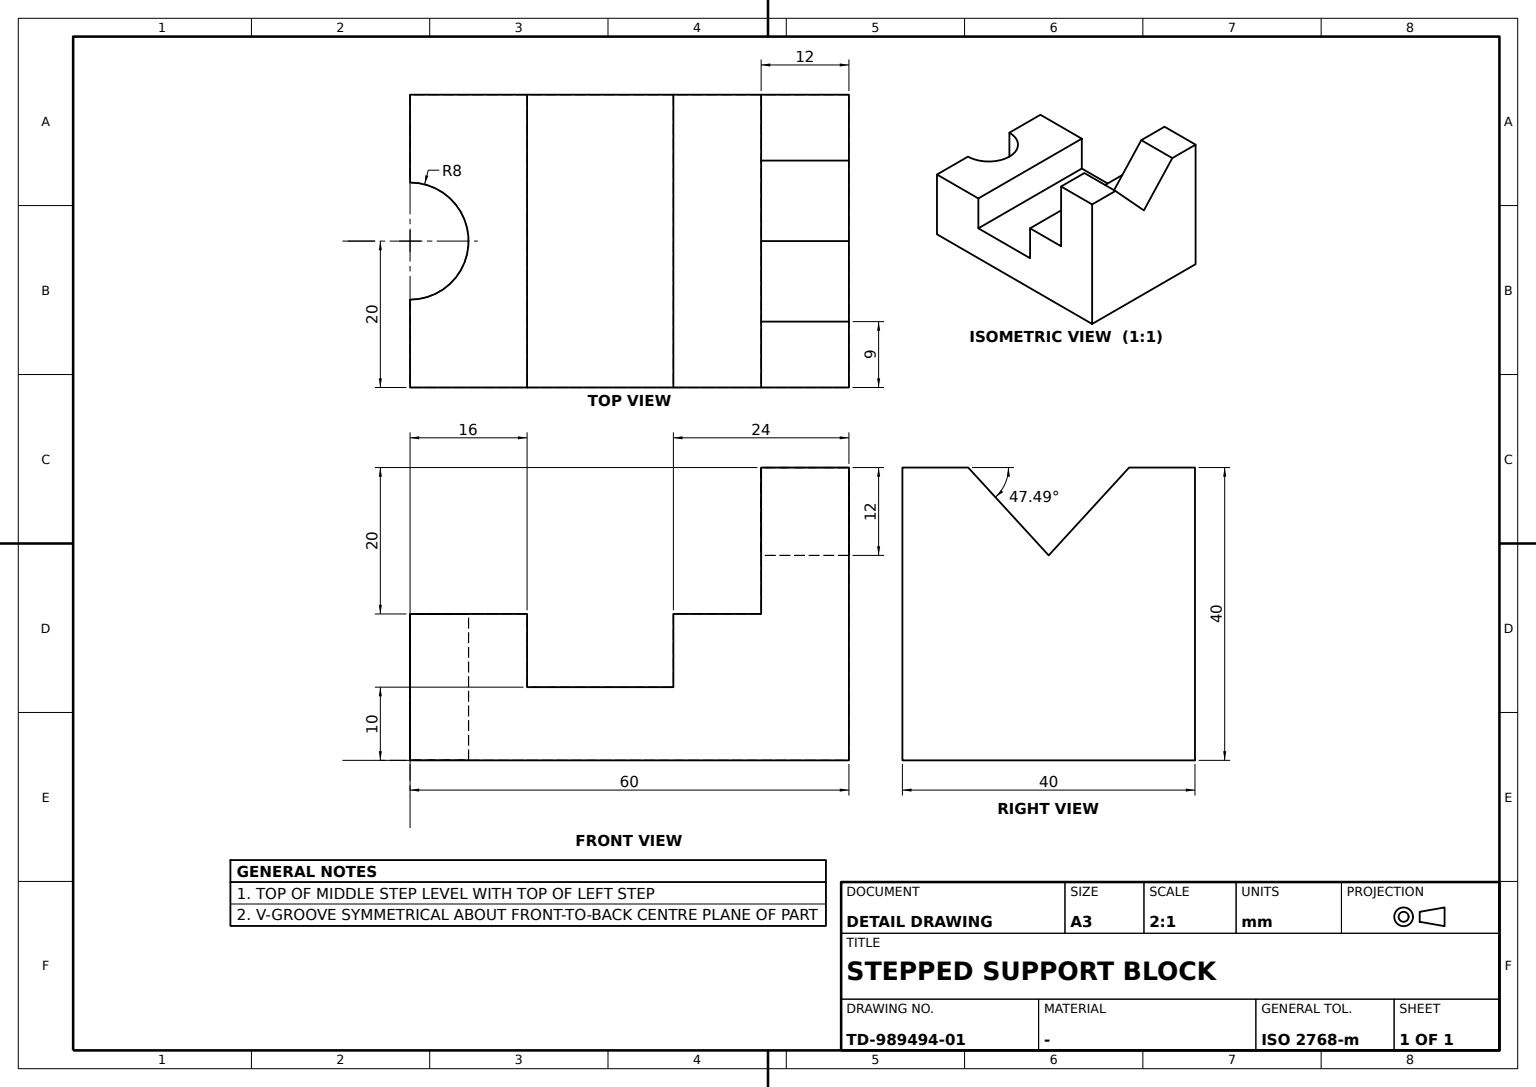
ISO-10303-21;
HEADER;
FILE_DESCRIPTION((''),'2;1');
FILE_NAME('','',(''),(''),'','','');
FILE_SCHEMA(('AUTOMOTIVE_DESIGN'));
ENDSEC;
DATA;
#1=APPLICATION_CONTEXT('');
#2=PRODUCT_CONTEXT('',#1,'mechanical');
#3=PRODUCT('','','',(#2));
#4=PRODUCT_DEFINITION_FORMATION('','',#3);
#5=PRODUCT_DEFINITION_CONTEXT('',#1,'design');
#6=PRODUCT_DEFINITION('','',#4,#5);
#7=PRODUCT_DEFINITION_SHAPE('','',#6);
#8=(LENGTH_UNIT()NAMED_UNIT(*)SI_UNIT(.MILLI.,.METRE.));
#9=(NAMED_UNIT(*)PLANE_ANGLE_UNIT()SI_UNIT($,.RADIAN.));
#10=(NAMED_UNIT(*)SI_UNIT($,.STERADIAN.)SOLID_ANGLE_UNIT());
#11=UNCERTAINTY_MEASURE_WITH_UNIT(LENGTH_MEASURE(0.005),#8,'distance_accuracy_value','');
#12=(GEOMETRIC_REPRESENTATION_CONTEXT(3)GLOBAL_UNCERTAINTY_ASSIGNED_CONTEXT((#11))GLOBAL_UNIT_ASSIGNED_CONTEXT((#8,#9,#10))REPRESENTATION_CONTEXT('',''));
#13=CARTESIAN_POINT('',(8.,0.,0.));
#14=VERTEX_POINT('',#13);
#15=CARTESIAN_POINT('',(20.,0.,0.));
#16=VERTEX_POINT('',#15);
#17=CARTESIAN_POINT('',(0.,0.,0.));
#18=DIRECTION('',(1.,0.,0.));
#19=VECTOR('',#18,1000.);
#20=LINE('',#17,#19);
#21=EDGE_CURVE('',#14,#16,#20,.T.);
#22=ORIENTED_EDGE('',*,*,#21,.T.);
#23=CARTESIAN_POINT('',(20.,0.,20.));
#24=VERTEX_POINT('',#23);
#25=DIRECTION('',(0.,0.,1.));
#26=VECTOR('',#25,1000.);
#27=LINE('',#15,#26);
#28=EDGE_CURVE('',#16,#24,#27,.T.);
#29=ORIENTED_EDGE('',*,*,#28,.T.);
#30=CARTESIAN_POINT('',(8.,0.,20.));
#31=VERTEX_POINT('',#30);
#32=CARTESIAN_POINT('',(0.,0.,20.));
#33=LINE('',#32,#19);
#34=EDGE_CURVE('',#31,#24,#33,.T.);
#35=ORIENTED_EDGE('',*,*,#34,.F.);
#36=LINE('',#13,#26);
#37=EDGE_CURVE('',#31,#14,#36,.F.);
#38=ORIENTED_EDGE('',*,*,#37,.T.);
#39=EDGE_LOOP('',(#22,#29,#35,#38));
#40=FACE_BOUND('',#39,.T.);
#41=DIRECTION('',(0.,1.,0.));
#42=AXIS2_PLACEMENT_3D('',#17,#41,#25);
#43=PLANE('',#42);
#44=ADVANCED_FACE('',(#40),#43,.F.);
#45=CARTESIAN_POINT('',(-8.,0.,20.));
#46=VERTEX_POINT('',#45);
#47=DIRECTION('',(0.,0.,-1.));
#48=DIRECTION('',(-1.,0.,0.));
#49=AXIS2_PLACEMENT_3D('',#32,#47,#48);
#50=CIRCLE('',#49,8.);
#51=EDGE_CURVE('',#31,#46,#50,.F.);
#52=ORIENTED_EDGE('',*,*,#51,.F.);
#53=ORIENTED_EDGE('',*,*,#34,.T.);
#54=CARTESIAN_POINT('',(20.,16.,20.));
#55=VERTEX_POINT('',#54);
#56=VECTOR('',#41,1000.);
#57=LINE('',#23,#56);
#58=EDGE_CURVE('',#24,#55,#57,.T.);
#59=ORIENTED_EDGE('',*,*,#58,.T.);
#60=CARTESIAN_POINT('',(-20.,16.,20.));
#61=VERTEX_POINT('',#60);
#62=CARTESIAN_POINT('',(0.,16.,20.));
#63=LINE('',#62,#19);
#64=EDGE_CURVE('',#61,#55,#63,.T.);
#65=ORIENTED_EDGE('',*,*,#64,.F.);
#66=CARTESIAN_POINT('',(-20.,0.,20.));
#67=VERTEX_POINT('',#66);
#68=LINE('',#66,#56);
#69=EDGE_CURVE('',#67,#61,#68,.T.);
#70=ORIENTED_EDGE('',*,*,#69,.F.);
#71=EDGE_CURVE('',#67,#46,#33,.T.);
#72=ORIENTED_EDGE('',*,*,#71,.T.);
#73=EDGE_LOOP('',(#52,#53,#59,#65,#70,#72));
#74=FACE_BOUND('',#73,.T.);
#75=CARTESIAN_POINT('',(0.,36.,20.));
#76=AXIS2_PLACEMENT_3D('',#75,#47,#41);
#77=PLANE('',#76);
#78=ADVANCED_FACE('',(#74),#77,.F.);
#79=CARTESIAN_POINT('',(-20.,16.,10.));
#80=VERTEX_POINT('',#79);
#81=CARTESIAN_POINT('',(20.,16.,10.));
#82=VERTEX_POINT('',#81);
#83=CARTESIAN_POINT('',(0.,16.,10.));
#84=LINE('',#83,#19);
#85=EDGE_CURVE('',#80,#82,#84,.T.);
#86=ORIENTED_EDGE('',*,*,#85,.F.);
#87=CARTESIAN_POINT('',(-20.,16.,0.));
#88=VECTOR('',#47,1000.);
#89=LINE('',#87,#88);
#90=EDGE_CURVE('',#61,#80,#89,.T.);
#91=ORIENTED_EDGE('',*,*,#90,.F.);
#92=ORIENTED_EDGE('',*,*,#64,.T.);
#93=CARTESIAN_POINT('',(20.,16.,0.));
#94=LINE('',#93,#88);
#95=EDGE_CURVE('',#55,#82,#94,.T.);
#96=ORIENTED_EDGE('',*,*,#95,.T.);
#97=EDGE_LOOP('',(#86,#91,#92,#96));
#98=FACE_BOUND('',#97,.T.);
#99=DIRECTION('',(0.,-1.,0.));
#100=AXIS2_PLACEMENT_3D('',#62,#99,#47);
#101=PLANE('',#100);
#102=ADVANCED_FACE('',(#98),#101,.F.);
#103=CARTESIAN_POINT('',(-20.,60.,0.));
#104=VERTEX_POINT('',#103);
#105=CARTESIAN_POINT('',(20.,60.,0.));
#106=VERTEX_POINT('',#105);
#107=CARTESIAN_POINT('',(0.,60.,0.));
#108=LINE('',#107,#19);
#109=EDGE_CURVE('',#104,#106,#108,.T.);
#110=ORIENTED_EDGE('',*,*,#109,.T.);
#111=VECTOR('',#99,1000.);
#112=LINE('',#15,#111);
#113=EDGE_CURVE('',#106,#16,#112,.T.);
#114=ORIENTED_EDGE('',*,*,#113,.T.);
#115=ORIENTED_EDGE('',*,*,#21,.F.);
#116=CARTESIAN_POINT('',(-8.,0.,0.));
#117=VERTEX_POINT('',#116);
#118=AXIS2_PLACEMENT_3D('',#17,#25,#18);
#119=CIRCLE('',#118,8.);
#120=EDGE_CURVE('',#14,#117,#119,.T.);
#121=ORIENTED_EDGE('',*,*,#120,.T.);
#122=CARTESIAN_POINT('',(-20.,0.,0.));
#123=VERTEX_POINT('',#122);
#124=EDGE_CURVE('',#123,#117,#20,.T.);
#125=ORIENTED_EDGE('',*,*,#124,.F.);
#126=LINE('',#122,#111);
#127=EDGE_CURVE('',#104,#123,#126,.T.);
#128=ORIENTED_EDGE('',*,*,#127,.F.);
#129=EDGE_LOOP('',(#110,#114,#115,#121,#125,#128));
#130=FACE_BOUND('',#129,.T.);
#131=AXIS2_PLACEMENT_3D('',#107,#25,#99);
#132=PLANE('',#131);
#133=ADVANCED_FACE('',(#130),#132,.F.);
#134=LINE('',#116,#26);
#135=EDGE_CURVE('',#117,#46,#134,.T.);
#136=ORIENTED_EDGE('',*,*,#135,.T.);
#137=ORIENTED_EDGE('',*,*,#71,.F.);
#138=LINE('',#122,#26);
#139=EDGE_CURVE('',#123,#67,#138,.T.);
#140=ORIENTED_EDGE('',*,*,#139,.F.);
#141=ORIENTED_EDGE('',*,*,#124,.T.);
#142=EDGE_LOOP('',(#136,#137,#140,#141));
#143=FACE_BOUND('',#142,.T.);
#144=ADVANCED_FACE('',(#143),#43,.F.);
#145=CARTESIAN_POINT('',(11.,60.,40.));
#146=VERTEX_POINT('',#145);
#147=CARTESIAN_POINT('',(11.,48.,40.));
#148=VERTEX_POINT('',#147);
#149=LINE('',#145,#111);
#150=EDGE_CURVE('',#146,#148,#149,.T.);
#151=ORIENTED_EDGE('',*,*,#150,.F.);
#152=CARTESIAN_POINT('',(0.,60.,28.));
#153=VERTEX_POINT('',#152);
#154=CARTESIAN_POINT('',(5.977358,60.,34.520755));
#155=DIRECTION('',(-0.675724629,0.,-0.73715414));
#156=VECTOR('',#155,1000.);
#157=LINE('',#154,#156);
#158=EDGE_CURVE('',#146,#153,#157,.T.);
#159=ORIENTED_EDGE('',*,*,#158,.T.);
#160=CARTESIAN_POINT('',(0.,48.,28.));
#161=VERTEX_POINT('',#160);
#162=LINE('',#152,#111);
#163=EDGE_CURVE('',#153,#161,#162,.T.);
#164=ORIENTED_EDGE('',*,*,#163,.T.);
#165=LINE('',#147,#156);
#166=EDGE_CURVE('',#148,#161,#165,.T.);
#167=ORIENTED_EDGE('',*,*,#166,.F.);
#168=EDGE_LOOP('',(#151,#159,#164,#167));
#169=FACE_BOUND('',#168,.T.);
#170=DIRECTION('',(-0.73715414,0.,0.675724629));
#171=AXIS2_PLACEMENT_3D('',#145,#170,#155);
#172=PLANE('',#171);
#173=ADVANCED_FACE('',(#169),#172,.T.);
#174=CARTESIAN_POINT('',(-20.,48.,40.));
#175=VERTEX_POINT('',#174);
#176=CARTESIAN_POINT('',(-20.,60.,40.));
#177=VERTEX_POINT('',#176);
#178=CARTESIAN_POINT('',(-20.,0.,40.));
#179=LINE('',#178,#56);
#180=EDGE_CURVE('',#175,#177,#179,.T.);
#181=ORIENTED_EDGE('',*,*,#180,.T.);
#182=LINE('',#103,#88);
#183=EDGE_CURVE('',#177,#104,#182,.T.);
#184=ORIENTED_EDGE('',*,*,#183,.T.);
#185=ORIENTED_EDGE('',*,*,#127,.T.);
#186=ORIENTED_EDGE('',*,*,#139,.T.);
#187=ORIENTED_EDGE('',*,*,#69,.T.);
#188=ORIENTED_EDGE('',*,*,#90,.T.);
#189=CARTESIAN_POINT('',(-20.,36.,10.));
#190=VERTEX_POINT('',#189);
#191=CARTESIAN_POINT('',(-20.,0.,10.));
#192=LINE('',#191,#56);
#193=EDGE_CURVE('',#80,#190,#192,.T.);
#194=ORIENTED_EDGE('',*,*,#193,.T.);
#195=CARTESIAN_POINT('',(-20.,36.,20.));
#196=VERTEX_POINT('',#195);
#197=CARTESIAN_POINT('',(-20.,36.,0.));
#198=LINE('',#197,#26);
#199=EDGE_CURVE('',#190,#196,#198,.T.);
#200=ORIENTED_EDGE('',*,*,#199,.T.);
#201=CARTESIAN_POINT('',(-20.,48.,20.));
#202=VERTEX_POINT('',#201);
#203=EDGE_CURVE('',#196,#202,#68,.T.);
#204=ORIENTED_EDGE('',*,*,#203,.T.);
#205=CARTESIAN_POINT('',(-20.,48.,0.));
#206=LINE('',#205,#26);
#207=EDGE_CURVE('',#202,#175,#206,.T.);
#208=ORIENTED_EDGE('',*,*,#207,.T.);
#209=EDGE_LOOP('',(#181,#184,#185,#186,#187,#188,#194,#200,#204,#208));
#210=FACE_BOUND('',#209,.T.);
#211=AXIS2_PLACEMENT_3D('',#122,#18,#41);
#212=PLANE('',#211);
#213=ADVANCED_FACE('',(#210),#212,.F.);
#214=ORIENTED_EDGE('',*,*,#199,.F.);
#215=CARTESIAN_POINT('',(20.,36.,10.));
#216=VERTEX_POINT('',#215);
#217=CARTESIAN_POINT('',(0.,36.,10.));
#218=LINE('',#217,#19);
#219=EDGE_CURVE('',#190,#216,#218,.T.);
#220=ORIENTED_EDGE('',*,*,#219,.T.);
#221=CARTESIAN_POINT('',(20.,36.,20.));
#222=VERTEX_POINT('',#221);
#223=CARTESIAN_POINT('',(20.,36.,0.));
#224=LINE('',#223,#26);
#225=EDGE_CURVE('',#216,#222,#224,.T.);
#226=ORIENTED_EDGE('',*,*,#225,.T.);
#227=LINE('',#75,#19);
#228=EDGE_CURVE('',#196,#222,#227,.T.);
#229=ORIENTED_EDGE('',*,*,#228,.F.);
#230=EDGE_LOOP('',(#214,#220,#226,#229));
#231=FACE_BOUND('',#230,.T.);
#232=AXIS2_PLACEMENT_3D('',#217,#41,#25);
#233=PLANE('',#232);
#234=ADVANCED_FACE('',(#231),#233,.F.);
#235=ORIENTED_EDGE('',*,*,#109,.F.);
#236=ORIENTED_EDGE('',*,*,#183,.F.);
#237=CARTESIAN_POINT('',(-11.,60.,40.));
#238=VERTEX_POINT('',#237);
#239=CARTESIAN_POINT('',(0.,60.,40.));
#240=LINE('',#239,#19);
#241=EDGE_CURVE('',#177,#238,#240,.T.);
#242=ORIENTED_EDGE('',*,*,#241,.T.);
#243=CARTESIAN_POINT('',(-5.977358,60.,34.520755));
#244=DIRECTION('',(-0.675724629,0.,0.73715414));
#245=VECTOR('',#244,1000.);
#246=LINE('',#243,#245);
#247=EDGE_CURVE('',#153,#238,#246,.T.);
#248=ORIENTED_EDGE('',*,*,#247,.F.);
#249=ORIENTED_EDGE('',*,*,#158,.F.);
#250=CARTESIAN_POINT('',(20.,60.,40.));
#251=VERTEX_POINT('',#250);
#252=EDGE_CURVE('',#146,#251,#240,.T.);
#253=ORIENTED_EDGE('',*,*,#252,.T.);
#254=LINE('',#105,#88);
#255=EDGE_CURVE('',#251,#106,#254,.T.);
#256=ORIENTED_EDGE('',*,*,#255,.T.);
#257=EDGE_LOOP('',(#235,#236,#242,#248,#249,#253,#256));
#258=FACE_BOUND('',#257,.T.);
#259=AXIS2_PLACEMENT_3D('',#239,#99,#47);
#260=PLANE('',#259);
#261=ADVANCED_FACE('',(#258),#260,.F.);
#262=CARTESIAN_POINT('',(20.,48.,40.));
#263=VERTEX_POINT('',#262);
#264=CARTESIAN_POINT('',(20.,0.,40.));
#265=LINE('',#264,#56);
#266=EDGE_CURVE('',#263,#251,#265,.T.);
#267=ORIENTED_EDGE('',*,*,#266,.F.);
#268=CARTESIAN_POINT('',(20.,48.,20.));
#269=VERTEX_POINT('',#268);
#270=CARTESIAN_POINT('',(20.,48.,0.));
#271=LINE('',#270,#26);
#272=EDGE_CURVE('',#269,#263,#271,.T.);
#273=ORIENTED_EDGE('',*,*,#272,.F.);
#274=EDGE_CURVE('',#222,#269,#57,.T.);
#275=ORIENTED_EDGE('',*,*,#274,.F.);
#276=ORIENTED_EDGE('',*,*,#225,.F.);
#277=CARTESIAN_POINT('',(20.,0.,10.));
#278=LINE('',#277,#56);
#279=EDGE_CURVE('',#82,#216,#278,.T.);
#280=ORIENTED_EDGE('',*,*,#279,.F.);
#281=ORIENTED_EDGE('',*,*,#95,.F.);
#282=ORIENTED_EDGE('',*,*,#58,.F.);
#283=ORIENTED_EDGE('',*,*,#28,.F.);
#284=ORIENTED_EDGE('',*,*,#113,.F.);
#285=ORIENTED_EDGE('',*,*,#255,.F.);
#286=EDGE_LOOP('',(#267,#273,#275,#276,#280,#281,#282,#283,#284,#285));
#287=FACE_BOUND('',#286,.T.);
#288=AXIS2_PLACEMENT_3D('',#15,#18,#41);
#289=PLANE('',#288);
#290=ADVANCED_FACE('',(#287),#289,.T.);
#291=ORIENTED_EDGE('',*,*,#37,.F.);
#292=ORIENTED_EDGE('',*,*,#51,.T.);
#293=ORIENTED_EDGE('',*,*,#135,.F.);
#294=ORIENTED_EDGE('',*,*,#120,.F.);
#295=EDGE_LOOP('',(#291,#292,#293,#294));
#296=FACE_BOUND('',#295,.T.);
#297=CARTESIAN_POINT('',(0.,0.,9.34));
#298=AXIS2_PLACEMENT_3D('',#297,#25,#18);
#299=CYLINDRICAL_SURFACE('',#298,8.);
#300=ADVANCED_FACE('',(#296),#299,.F.);
#301=ORIENTED_EDGE('',*,*,#219,.F.);
#302=ORIENTED_EDGE('',*,*,#193,.F.);
#303=ORIENTED_EDGE('',*,*,#85,.T.);
#304=ORIENTED_EDGE('',*,*,#279,.T.);
#305=EDGE_LOOP('',(#301,#302,#303,#304));
#306=FACE_BOUND('',#305,.T.);
#307=AXIS2_PLACEMENT_3D('',#83,#47,#41);
#308=PLANE('',#307);
#309=ADVANCED_FACE('',(#306),#308,.F.);
#310=ORIENTED_EDGE('',*,*,#163,.F.);
#311=ORIENTED_EDGE('',*,*,#247,.T.);
#312=CARTESIAN_POINT('',(-11.,48.,40.));
#313=VERTEX_POINT('',#312);
#314=LINE('',#312,#111);
#315=EDGE_CURVE('',#238,#313,#314,.T.);
#316=ORIENTED_EDGE('',*,*,#315,.T.);
#317=CARTESIAN_POINT('',(3.984906,48.,23.65283));
#318=DIRECTION('',(0.675724629,0.,-0.73715414));
#319=VECTOR('',#318,1000.);
#320=LINE('',#317,#319);
#321=EDGE_CURVE('',#313,#161,#320,.T.);
#322=ORIENTED_EDGE('',*,*,#321,.T.);
#323=EDGE_LOOP('',(#310,#311,#316,#322));
#324=FACE_BOUND('',#323,.T.);
#325=DIRECTION('',(0.73715414,0.,0.675724629));
#326=AXIS2_PLACEMENT_3D('',#152,#325,#244);
#327=PLANE('',#326);
#328=ADVANCED_FACE('',(#324),#327,.T.);
#329=CARTESIAN_POINT('',(0.,48.,40.));
#330=LINE('',#329,#19);
#331=EDGE_CURVE('',#175,#313,#330,.T.);
#332=ORIENTED_EDGE('',*,*,#331,.T.);
#333=ORIENTED_EDGE('',*,*,#315,.F.);
#334=ORIENTED_EDGE('',*,*,#241,.F.);
#335=ORIENTED_EDGE('',*,*,#180,.F.);
#336=EDGE_LOOP('',(#332,#333,#334,#335));
#337=FACE_BOUND('',#336,.T.);
#338=AXIS2_PLACEMENT_3D('',#329,#47,#41);
#339=PLANE('',#338);
#340=ADVANCED_FACE('',(#337),#339,.F.);
#341=ORIENTED_EDGE('',*,*,#321,.F.);
#342=ORIENTED_EDGE('',*,*,#331,.F.);
#343=ORIENTED_EDGE('',*,*,#207,.F.);
#344=CARTESIAN_POINT('',(0.,48.,20.));
#345=LINE('',#344,#19);
#346=EDGE_CURVE('',#202,#269,#345,.T.);
#347=ORIENTED_EDGE('',*,*,#346,.T.);
#348=ORIENTED_EDGE('',*,*,#272,.T.);
#349=EDGE_CURVE('',#148,#263,#330,.T.);
#350=ORIENTED_EDGE('',*,*,#349,.F.);
#351=ORIENTED_EDGE('',*,*,#166,.T.);
#352=EDGE_LOOP('',(#341,#342,#343,#347,#348,#350,#351));
#353=FACE_BOUND('',#352,.T.);
#354=AXIS2_PLACEMENT_3D('',#344,#41,#25);
#355=PLANE('',#354);
#356=ADVANCED_FACE('',(#353),#355,.F.);
#357=ORIENTED_EDGE('',*,*,#252,.F.);
#358=ORIENTED_EDGE('',*,*,#150,.T.);
#359=ORIENTED_EDGE('',*,*,#349,.T.);
#360=ORIENTED_EDGE('',*,*,#266,.T.);
#361=EDGE_LOOP('',(#357,#358,#359,#360));
#362=FACE_BOUND('',#361,.T.);
#363=ADVANCED_FACE('',(#362),#339,.F.);
#364=ORIENTED_EDGE('',*,*,#228,.T.);
#365=ORIENTED_EDGE('',*,*,#274,.T.);
#366=ORIENTED_EDGE('',*,*,#346,.F.);
#367=ORIENTED_EDGE('',*,*,#203,.F.);
#368=EDGE_LOOP('',(#364,#365,#366,#367));
#369=FACE_BOUND('',#368,.T.);
#370=ADVANCED_FACE('',(#369),#77,.F.);
#371=CLOSED_SHELL('',(#44,#78,#102,#133,#144,#173,#213,#234,#261,#290,#300,#309,#328,#340,#356,#363,#370));
#372=MANIFOLD_SOLID_BREP('',#371);
#373=ADVANCED_BREP_SHAPE_REPRESENTATION('',(#372),#12);
#374=SHAPE_DEFINITION_REPRESENTATION(#7,#373);
ENDSEC;
END-ISO-10303-21;
